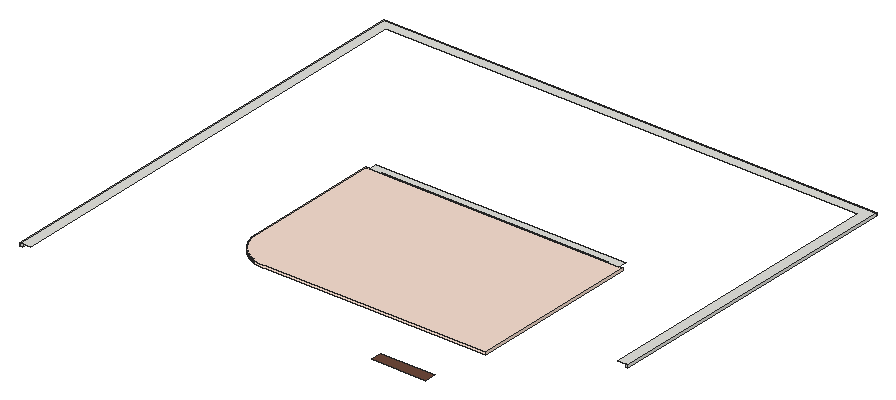
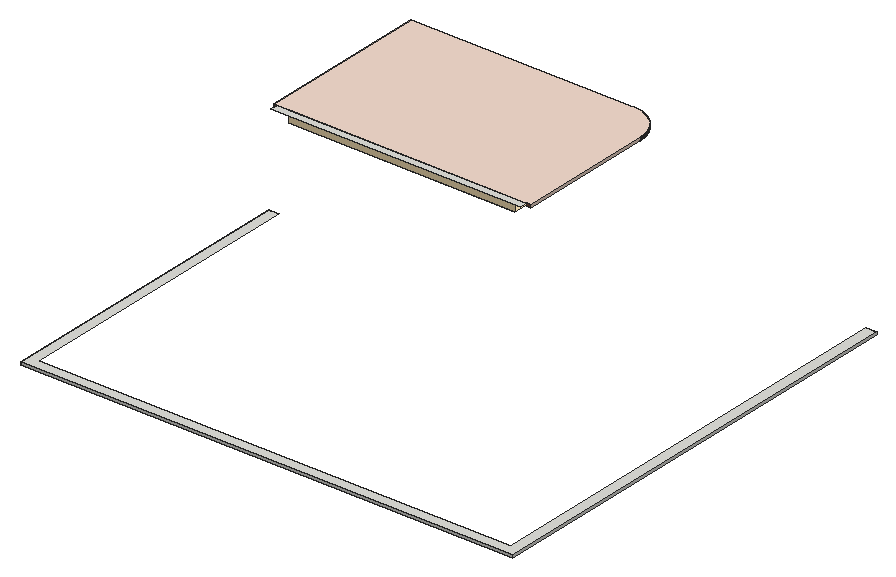
# SketchUp Ruby script. Lengths in inches.
U = 1.inch
M = Sketchup.active_model
def pt(a) = Geom::Point3d.new(a.map { |v| v * U })
def face(e, loops, mat)
  f = e.add_face(loops[0].map { |a| pt(a) })
  loops[1..].each { |l| e.add_face(l.map { |a| pt(a) }).erase! }
  f.material = f.back_material = mat if mat
  f
end
# faces: each face lists its corners as indices into pts; further lists are holes
def faces(e, pts, list, mat = nil) = list.each { |f| face(e, (f[0].is_a?(Array) ? f : [f]).map { |l| l.map { |i| pts[i] } }, mat) }
# xy, xz, yz: faces in a plane at the given z, y or x. An outline is a flat list of corners, or four numbers for a rectangle; further outlines are holes
def ring(l) = l.size == 4 ? [[l[0], l[1]], [l[2], l[1]], [l[2], l[3]], [l[0], l[3]]] : l.each_slice(2).to_a
def flat(e, list, mat, &to3) = list.each { |f| face(e, (f[0].is_a?(Array) ? f : [f]).map { |l| ring(l).map { |u, v| to3.(u, v) } }, mat) }
def xy(e, z, list, mat = nil) = flat(e, list, mat) { |x, y| [x, y, z] }
def xz(e, y, list, mat = nil) = flat(e, list, mat) { |x, z| [x, y, z] }
def yz(e, x, list, mat = nil) = flat(e, list, mat) { |y, z| [x, y, z] }
def lines(e, pts, list) = list.each { |a, b| e.add_line(pt(pts[a]), pt(pts[b])) }
# prism: a flat outline (further loops are holes) pulled along v
def prism(e, loops, v, mat = nil)
  f = face(e, loops, mat); d = Geom::Vector3d.new(v.map { |x| x * U })
  f.pushpull(f.normal.samedirection?(d) ? d.length : -d.length)
end
def box(e, o, s, mat = nil) = prism(e, [[o, [o[0] + s[0], o[1], o[2]], [o[0] + s[0], o[1] + s[1], o[2]], [o[0], o[1] + s[1], o[2]]]], [0, 0, s[2]], mat)
def at(x, y, z, deg = 0) = Geom::Transformation.translation(pt([x, y, z])) * Geom::Transformation.rotation(ORIGIN, Z_AXIS, deg.degrees)
def axes(o, x, y, z) = Geom::Transformation.new([*x, 0, *y, 0, *z, 0, *pt(o).to_a, 1])
def part(name) = M.definitions.add(name)
# library, detail: a bought-in or finely detailed component or shape, given as its bounding box
def library(name, o, s) = part(name).tap { |d| box(d.entities, o, s) }
def detail(e, o, s) = box(e.add_group.entities, o, s)
def put(e, d, t, mat = nil) = e.add_instance(d, t).tap { |i| i.material = mat if mat }
def group(e, t, mat = nil) = e.add_group.tap { |g| g.transformation = t; g.material = mat if mat }.entities
root = M.entities
M.materials.add("1026 AP 7946 SUNNY SIDE UP").color = [254, 231, 186]
M.materials.add("1916 AP K226 Macadamia Cream-N").color = [109, 72, 58]
M.materials.add("1937 AP K247 Camellia Bud-N").color = [246, 221, 207]
xy(root,300,[[16,326.09,16,676,395,676,395,437,393,437,393,674,18,674,18,326.09]])
xy(root,302,[[16,326.09,24,326.09,24,668,387,668,387,437,395,437,395,676,16,676]])
xy(root,333.89,[[305.52,302,347.52,311]],"1916 AP K226 Macadamia Cream-N")
xy(root,363,[[224.71,311,224.56,311.01,224.41,311.01,224.26,311.02,224.12,311.03,223.82,311.05,223.68,311.06,223.53,311.07,223.38,311.09,223.24,311.1,222.94,311.14,222.8,311.16,222.65,311.18,222.51,311.21,222.36,311.23,222.22,311.26,222.07,311.29,221.79,311.35,221.64,311.38,221.5,311.41,221.36,311.45,221.21,311.49,221.07,311.52,220.93,311.5625,220.79,311.6,220.65,311.65,220.51,311.6875,220.36,311.73,220.22,311.78,220.09,311.83,219.95,311.875,219.81,311.93,219.53,312.03,219.4,312.09,219.26,312.14,218.99,312.26,218.85,312.32,218.59,312.44,218.45,312.5,218.32,312.57,218.19,312.63,217.67,312.91,217.54,312.99,217.42,313.06,217.29,313.13,217.16,313.21,217.04,313.29,216.91,313.37,216.67,313.53,216.54,313.61,216.42,313.69,216.3,313.78,216.18,313.86,216.06,313.95,215.95,314.04,215.71,314.22,215.6,314.3125,215.48,314.4,215.37,314.5,215.26,314.59,214.71,315.09,214.6,315.1875,214.5,315.29,214.39,315.39,214.29,315.5,214.1875,315.6,214.09,315.71,213.59,316.26,213.5,316.37,213.4,316.48,213.3125,316.6,213.22,316.71,213.04,316.95,212.95,317.06,212.86,317.18,212.78,317.3,212.69,317.42,212.61,317.54,212.53,317.67,212.37,317.91,212.29,318.04,212.21,318.16,212.13,318.29,212.06,318.42,211.99,318.54,211.91,318.67,211.63,319.19,211.57,319.32,211.5,319.45,211.44,319.59,211.32,319.85,211.26,319.99,211.14,320.26,211.09,320.4,211.03,320.53,210.93,320.81,210.875,320.95,210.83,321.09,210.78,321.22,210.73,321.36,210.6875,321.51,210.65,321.65,210.6,321.79,210.5625,321.93,210.52,322.07,210.49,322.21,210.45,322.36,210.41,322.5,210.38,322.64,210.35,322.79,210.29,323.07,210.26,323.22,210.23,323.36,210.21,323.51,210.18,323.65,210.16,323.8,210.14,323.94,210.1,324.24,210.09,324.38,210.07,324.53,210.06,324.68,210.05,324.82,210.03,325.12,210.02,325.26,210.01,325.41,210.01,325.56,210,325.71,210,431,384,431,384,311]],"1026 AP 7946 SUNNY SIDE UP")
xy(root,370,[[224.73,299,224.47,299.01,224.2,299.01,223.68,299.03,223.41,299.05,223.15,299.0625,222.88,299.08,222.62,299.11,222.35,299.13,222.09,299.16,221.83,299.1875,221.5625,299.22,221.3,299.25,220.78,299.33,220.51,299.375,220.25,299.42,219.47,299.57,219.21,299.63,218.96,299.69,218.44,299.81,218.18,299.875,217.93,299.94,217.67,300.01,217.42,300.09,217.16,300.16,216.66,300.32,216.4,300.4,215.65,300.67,215.41,300.76,214.91,300.96,214.67,301.06,214.42,301.16,214.18,301.26,213.9375,301.37,213.7,301.48,213.46,301.59,213.22,301.71,212.98,301.82,212.74,301.94,212.51,302.0625,212.27,302.1875,212.04,302.3125,211.81,302.44,211.58,302.57,211.35,302.71,211.12,302.84,210.89,302.98,210.67,303.12,210.44,303.26,210.22,303.4,209.78,303.7,209.5625,303.85,209.35,304,209.13,304.16,208.92,304.3125,208.7,304.47,208.49,304.63,208.28,304.8,208.08,304.96,207.87,305.13,207.67,305.3,207.46,305.47,207.26,305.64,207.07,305.82,206.87,305.99,206.67,306.17,206.48,306.35,206.29,306.54,206.1,306.72,205.72,307.1,205.54,307.29,205.35,307.48,205.17,307.67,204.99,307.87,204.82,308.07,204.64,308.26,204.47,308.46,204.3,308.67,204.13,308.87,203.96,309.08,203.8,309.28,203.63,309.49,203.47,309.7,203.3125,309.92,203.16,310.13,203,310.35,202.85,310.5625,202.7,310.78,202.4,311.22,202.26,311.44,202.12,311.67,201.98,311.89,201.84,312.12,201.71,312.35,201.57,312.58,201.44,312.81,201.3125,313.04,201.1875,313.27,201.0625,313.51,200.94,313.74,200.82,313.98,200.71,314.22,200.59,314.46,200.48,314.7,200.37,314.9375,200.26,315.18,200.16,315.42,200.06,315.67,199.96,315.91,199.76,316.41,199.67,316.65,199.4,317.4,199.32,317.66,199.16,318.16,199.09,318.42,199.01,318.67,198.94,318.93,198.875,319.18,198.81,319.44,198.69,319.96,198.63,320.21,198.57,320.47,198.42,321.25,198.375,321.51,198.33,321.78,198.25,322.3,198.22,322.5625,198.1875,322.83,198.16,323.09,198.13,323.35,198.11,323.62,198.08,323.88,198.0625,324.15,198.05,324.41,198.03,324.68,198.01,325.2,198.01,325.47,198,325.73,198,431,201,431,201,325.53,201.01,325.29,201.02,325.06,201.03,324.82,201.04,324.59,201.06,324.35,201.07,324.12,201.09,323.88,201.12,323.65,201.14,323.41,201.2,322.95,201.23,322.71,201.26,322.48,201.3,322.25,201.33,322.01,201.42,321.55,201.46,321.32,201.56,320.86,201.61,320.625,201.66,320.4,201.84,319.71,201.9,319.49,201.97,319.26,202.03,319.03,202.1,318.81,202.17,318.58,202.25,318.36,202.32,318.14,202.4,317.91,202.48,317.69,202.57,317.47,202.65,317.25,202.74,317.03,202.83,316.82,203.01,316.38,203.11,316.17,203.2,315.95,203.3,315.74,203.41,315.53,203.51,315.31,203.62,315.1,203.72,314.89,203.83,314.6875,203.95,314.48,204.06,314.27,204.18,314.07,204.29,313.86,204.41,313.66,204.54,313.46,204.66,313.26,204.79,313.0625,204.91,312.86,205.04,312.67,205.18,312.47,205.31,312.28,205.45,312.08,205.58,311.89,205.86,311.51,206.01,311.33,206.15,311.14,206.3,310.96,206.45,310.77,206.9,310.23,207.06,310.06,207.22,309.88,207.375,309.71,207.54,309.54,207.86,309.2,208.2,308.86,208.54,308.54,208.71,308.375,208.88,308.22,209.06,308.06,209.23,307.9,209.77,307.45,209.96,307.3,210.14,307.15,210.33,307.01,210.51,306.86,210.89,306.58,211.08,306.45,211.28,306.31,211.47,306.18,211.67,306.04,211.86,305.91,212.0625,305.79,212.26,305.66,212.46,305.54,212.66,305.41,212.86,305.29,213.07,305.18,213.27,305.06,213.48,304.95,213.6875,304.83,213.89,304.72,214.1,304.62,214.31,304.51,214.53,304.41,214.74,304.3,214.95,304.2,215.17,304.11,215.38,304.01,215.82,303.83,216.03,303.74,216.25,303.65,216.47,303.57,216.69,303.48,216.91,303.4,217.14,303.32,217.36,303.25,217.58,303.17,217.81,303.1,218.03,303.03,218.26,302.97,218.49,302.9,218.71,302.84,219.4,302.66,219.625,302.61,219.86,302.56,220.32,302.46,220.55,302.42,221.01,302.33,221.25,302.3,221.48,302.26,221.71,302.23,221.95,302.2,222.41,302.14,222.65,302.12,222.88,302.09,223.12,302.07,223.35,302.06,223.59,302.04,223.82,302.03,224.06,302.02,224.29,302.01,224.53,302,393,302,393,431,396,431,396,299]],"1937 AP K247 Camellia Bud-N")
xy(root,372,[[201,431,393,437]])
xy(root,372,[[224.73,299,396,299,396,431,198,431,198,325.73,198.01,325.47,198.01,325.2,198.03,324.68,198.05,324.41,198.0625,324.15,198.08,323.88,198.11,323.62,198.13,323.35,198.16,323.09,198.1875,322.83,198.22,322.5625,198.25,322.3,198.33,321.78,198.375,321.51,198.42,321.25,198.57,320.47,198.63,320.21,198.69,319.96,198.81,319.44,198.875,319.18,198.94,318.93,199.01,318.67,199.09,318.42,199.16,318.16,199.32,317.66,199.4,317.4,199.67,316.65,199.76,316.41,199.96,315.91,200.06,315.67,200.16,315.42,200.26,315.18,200.37,314.9375,200.48,314.7,200.59,314.46,200.71,314.22,200.82,313.98,200.94,313.74,201.0625,313.51,201.1875,313.27,201.3125,313.04,201.44,312.81,201.57,312.58,201.71,312.35,201.84,312.12,201.98,311.89,202.12,311.67,202.26,311.44,202.4,311.22,202.7,310.78,202.85,310.5625,203,310.35,203.16,310.13,203.3125,309.92,203.47,309.7,203.63,309.49,203.8,309.28,203.96,309.08,204.13,308.87,204.3,308.67,204.47,308.46,204.64,308.26,204.82,308.07,204.99,307.87,205.17,307.67,205.35,307.48,205.54,307.29,205.72,307.1,206.1,306.72,206.29,306.54,206.48,306.35,206.67,306.17,206.87,305.99,207.07,305.82,207.26,305.64,207.46,305.47,207.67,305.3,207.87,305.13,208.08,304.96,208.28,304.8,208.49,304.63,208.7,304.47,208.92,304.3125,209.13,304.16,209.35,304,209.5625,303.85,209.78,303.7,210.22,303.4,210.44,303.26,210.67,303.12,210.89,302.98,211.12,302.84,211.35,302.71,211.58,302.57,211.81,302.44,212.04,302.3125,212.27,302.1875,212.51,302.0625,212.74,301.94,212.98,301.82,213.22,301.71,213.46,301.59,213.7,301.48,213.9375,301.37,214.18,301.26,214.42,301.16,214.67,301.06,214.91,300.96,215.41,300.76,215.65,300.67,216.4,300.4,216.66,300.32,217.16,300.16,217.42,300.09,217.67,300.01,217.93,299.94,218.18,299.875,218.44,299.81,218.96,299.69,219.21,299.63,219.47,299.57,220.25,299.42,220.51,299.375,220.78,299.33,221.3,299.25,221.5625,299.22,221.83,299.1875,222.09,299.16,222.35,299.13,222.62,299.11,222.88,299.08,223.15,299.0625,223.41,299.05,223.68,299.03,224.2,299.01,224.47,299.01]],"1937 AP K247 Camellia Bud-N")
xz(root,326.09,[[16,300,18,302]])
xz(root,431,[[210,363,384,372]],"1026 AP 7946 SUNNY SIDE UP")
xz(root,431,[[198,370,201,372],[393,370,396,372]],"1916 AP K226 Macadamia Cream-N")
xz(root,437,[[393,300,395,302]])
xz(root,676,[[16,300,395,302]])
yz(root,16,[[326.09,300,676,302]])
yz(root,198,[[325.73,370,326,372],[326,370,431,372]],"1937 AP K247 Camellia Bud-N")
yz(root,198.01,[[325.2,370,325.47,372]],"1937 AP K247 Camellia Bud-N")
yz(root,395,[[437,300,676,302]])
yz(root,396,[[299,370,431,372]],"1937 AP K247 Camellia Bud-N")
p = [[216.66,300.32,372],[216.4,300.4,372],[216.4,300.4,370],[216.66,300.32,370],[216.15,300.49,372],[216.15,300.49,370],
  [215.9,300.58,372],[215.9,300.58,370],[215.65,300.67,372],[215.65,300.67,370],[215.41,300.76,372],[215.41,300.76,370],
  [215.16,300.86,372],[215.16,300.86,370],[214.91,300.96,372],[214.91,300.96,370],[214.67,301.06,372],[214.67,301.06,370],
  [214.42,301.16,372],[214.42,301.16,370],[214.18,301.26,372],[214.18,301.26,370],[213.9375,301.37,372],[213.9375,301.37,370],
  [213.7,301.48,372],[213.7,301.48,370],[213.46,301.59,372],[213.46,301.59,370],[213.22,301.71,372],[213.22,301.71,370],
  [212.98,301.82,372],[212.98,301.82,370],[212.74,301.94,372],[212.74,301.94,370],[212.51,302.0625,372],[212.51,302.0625,370],
  [212.27,302.1875,372],[212.27,302.1875,370],[212.04,302.3125,372],[212.04,302.3125,370],[211.81,302.44,372],[211.81,302.44,370],
  [211.58,302.57,372],[211.58,302.57,370],[211.35,302.71,372],[211.35,302.71,370],[211.12,302.84,372],[211.12,302.84,370],
  [210.89,302.98,372],[210.89,302.98,370],[210.67,303.12,372],[210.67,303.12,370],[210.44,303.26,372],[210.44,303.26,370],
  [210.22,303.4,372],[210.22,303.4,370],[210,303.55,372],[210,303.55,370],[209.78,303.7,372],[209.78,303.7,370],
  [209.5625,303.85,372],[209.5625,303.85,370],[209.35,304,372],[209.35,304,370],[209.13,304.16,372],[209.13,304.16,370],
  [208.92,304.3125,372],[208.92,304.3125,370],[208.7,304.47,372],[208.7,304.47,370],[208.49,304.63,372],[208.49,304.63,370],
  [208.28,304.8,372],[208.28,304.8,370],[208.08,304.96,372],[208.08,304.96,370],[207.87,305.13,372],[207.87,305.13,370],
  [207.67,305.3,372],[207.67,305.3,370],[207.46,305.47,372],[207.46,305.47,370],[207.26,305.64,372],[207.26,305.64,370],
  [207.07,305.82,372],[207.07,305.82,370],[206.87,305.99,372],[206.87,305.99,370],[206.67,306.17,372],[206.67,306.17,370],
  [206.48,306.35,372],[206.48,306.35,370],[206.29,306.54,372],[206.29,306.54,370],[206.1,306.72,372],[206.1,306.72,370],
  [205.91,306.91,372],[205.91,306.91,370],[205.72,307.1,372],[205.72,307.1,370],[205.54,307.29,372],[205.54,307.29,370],
  [205.35,307.48,372],[205.35,307.48,370],[205.17,307.67,372],[205.17,307.67,370],[204.99,307.87,372],[204.99,307.87,370],
  [204.82,308.07,372],[204.82,308.07,370],[204.64,308.26,372],[204.64,308.26,370],[204.47,308.46,372],[204.47,308.46,370],
  [204.3,308.67,372],[204.3,308.67,370],[204.13,308.87,372],[204.13,308.87,370],[203.96,309.08,372],[203.96,309.08,370],
  [203.8,309.28,372],[203.8,309.28,370],[203.63,309.49,372],[203.63,309.49,370],[203.47,309.7,372],[203.47,309.7,370],
  [203.3125,309.92,372],[203.3125,309.92,370],[203.16,310.13,372],[203.16,310.13,370],[203,310.35,372],[203,310.35,370],
  [202.85,310.5625,372],[202.85,310.5625,370],[202.7,310.78,372],[202.7,310.78,370],[202.55,311,372],[202.55,311,370],
  [202.4,311.22,372],[202.4,311.22,370],[202.26,311.44,372],[202.26,311.44,370],[202.12,311.67,372],[202.12,311.67,370],
  [201.98,311.89,372],[201.98,311.89,370],[201.84,312.12,372],[201.84,312.12,370],[201.71,312.35,372],[201.71,312.35,370],
  [201.57,312.58,372],[201.57,312.58,370],[201.44,312.81,372],[201.44,312.81,370],[201.3125,313.04,372],[201.3125,313.04,370],
  [201.1875,313.27,372],[201.1875,313.27,370],[201.0625,313.51,372],[201.0625,313.51,370],[200.94,313.74,372],[200.94,313.74,370],
  [200.82,313.98,372],[200.82,313.98,370],[200.71,314.22,372],[200.71,314.22,370],[200.59,314.46,372],[200.59,314.46,370],
  [200.48,314.7,372],[200.48,314.7,370],[200.37,314.9375,372],[200.37,314.9375,370],[200.26,315.18,372],[200.26,315.18,370],
  [200.16,315.42,372],[200.16,315.42,370],[200.06,315.67,372],[200.06,315.67,370],[199.96,315.91,372],[199.96,315.91,370],
  [199.86,316.16,372],[199.86,316.16,370],[199.76,316.41,372],[199.76,316.41,370],[199.67,316.65,372],[199.67,316.65,370],
  [199.58,316.9,372],[199.58,316.9,370],[199.49,317.15,372],[199.49,317.15,370],[199.4,317.4,372],[199.4,317.4,370],
  [199.32,317.66,372],[199.32,317.66,370],[199.24,317.91,372],[199.24,317.91,370],[199.16,318.16,372],[199.16,318.16,370],
  [199.09,318.42,372],[199.09,318.42,370],[199.01,318.67,372],[199.01,318.67,370],[198.94,318.93,372],[198.94,318.93,370],
  [198.875,319.18,372],[198.875,319.18,370],[198.81,319.44,372],[198.81,319.44,370],[198.75,319.7,372],[198.75,319.7,370],
  [198.69,319.96,372],[198.69,319.96,370],[198.63,320.21,372],[198.63,320.21,370],[198.57,320.47,372],[198.57,320.47,370],
  [198.52,320.73,372],[198.52,320.73,370],[198.47,320.99,372],[198.47,320.99,370],[198.42,321.25,372],[198.42,321.25,370],
  [198.375,321.51,372],[198.375,321.51,370],[198.33,321.78,372],[198.33,321.78,370],[198.29,322.04,372],[198.29,322.04,370],
  [198.25,322.3,372],[198.25,322.3,370],[198.22,322.5625,372],[198.22,322.5625,370],[198.1875,322.83,372],[198.1875,322.83,370],
  [198.16,323.09,372],[198.16,323.09,370],[198.13,323.35,372],[198.13,323.35,370],[198.11,323.62,372],[198.11,323.62,370],
  [198.08,323.88,372],[198.08,323.88,370],[198.0625,324.15,372],[198.0625,324.15,370],[198.05,324.41,372],[198.05,324.41,370],
  [198.03,324.68,372],[198.03,324.68,370],[198.02,324.94,372],[198.02,324.94,370],[198.01,325.2,372],[198.01,325.2,370],
  [198.01,325.47,372],[198,325.73,372],[198,325.73,370],[198.01,325.47,370],[198,431,372],[197.6875,431,372],
  [224.85,302,372],[225,302,372],[393,674,300],[393,674,302],[18,674,300],[18,674,302]]
faces(root,p,[[0,1,2,3],[1,4,5,2],[4,6,7,5],[6,8,9,7],[8,10,11,9],[10,12,13,11],[12,14,15,13],[14,16,17,15],
  [16,18,19,17],[18,20,21,19],[20,22,23,21],[22,24,25,23],[24,26,27,25],[26,28,29,27],[28,30,31,29],[30,32,33,31],
  [32,34,35,33],[34,36,37,35],[36,38,39,37],[38,40,41,39],[40,42,43,41],[42,44,45,43],[44,46,47,45],[46,48,49,47],
  [48,50,51,49],[50,52,53,51],[52,54,55,53],[54,56,57,55],[56,58,59,57],[58,60,61,59],[60,62,63,61],[62,64,65,63],
  [64,66,67,65],[66,68,69,67],[68,70,71,69],[70,72,73,71],[72,74,75,73],[74,76,77,75],[76,78,79,77],[78,80,81,79],
  [80,82,83,81],[82,84,85,83],[84,86,87,85],[86,88,89,87],[88,90,91,89],[90,92,93,91],[92,94,95,93],[94,96,97,95],
  [96,98,99,97],[98,100,101,99],[100,102,103,101],[102,104,105,103],[104,106,107,105],[106,108,109,107],[108,110,111,109],[110,112,113,111],
  [112,114,115,113],[114,116,117,115],[116,118,119,117],[118,120,121,119],[120,122,123,121],[122,124,125,123],[124,126,127,125],[126,128,129,127],
  [128,130,131,129],[130,132,133,131],[132,134,135,133],[134,136,137,135],[136,138,139,137],[138,140,141,139],[140,142,143,141],[142,144,145,143],
  [144,146,147,145],[146,148,149,147],[148,150,151,149],[150,152,153,151],[152,154,155,153],[154,156,157,155],[156,158,159,157],[158,160,161,159],
  [160,162,163,161],[162,164,165,163],[164,166,167,165],[166,168,169,167],[168,170,171,169],[170,172,173,171],[172,174,175,173],[174,176,177,175],
  [176,178,179,177],[178,180,181,179],[180,182,183,181],[182,184,185,183],[184,186,187,185],[186,188,189,187],[188,190,191,189],[190,192,193,191],
  [192,194,195,193],[194,196,197,195],[196,198,199,197],[198,200,201,199],[200,202,203,201],[202,204,205,203],[204,206,207,205],[206,208,209,207],
  [208,210,211,209],[210,212,213,211],[212,214,215,213],[214,216,217,215],[216,218,219,217],[218,220,221,219],[220,222,223,221],[222,224,225,223],
  [224,226,227,225],[226,228,229,227],[228,230,231,229],[230,232,233,231],[232,234,235,233],[234,236,237,235],[236,238,239,237],[238,240,241,239],
  [240,242,243,241],[242,244,245,243],[244,246,247,245],[246,248,249,247],[248,250,251,249],[252,253,254,255]],"1937 AP K247 Camellia Bud-N")
lines(root,p,[[256,257],[258,259],[260,261],[262,263]])
